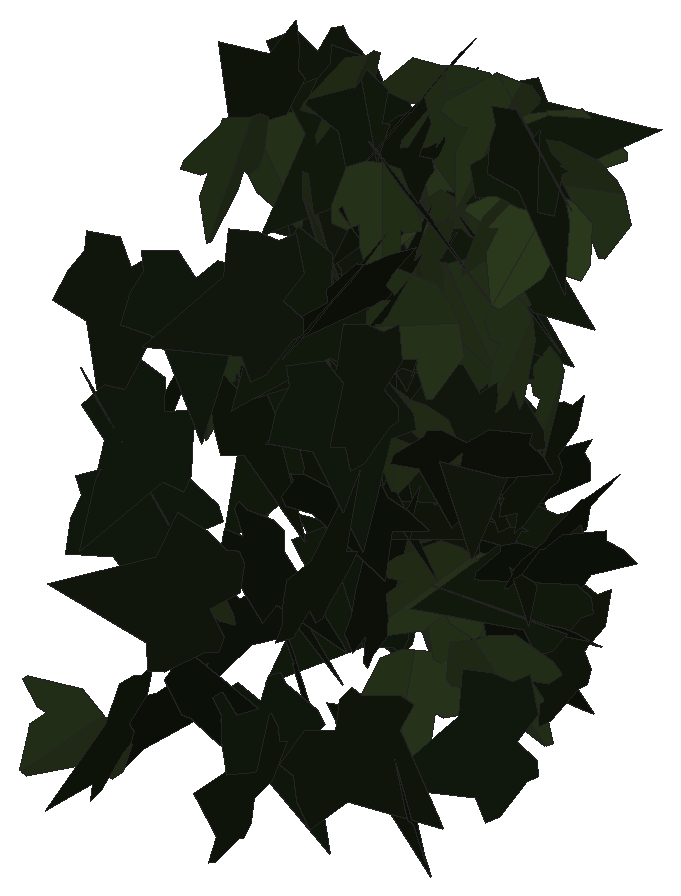
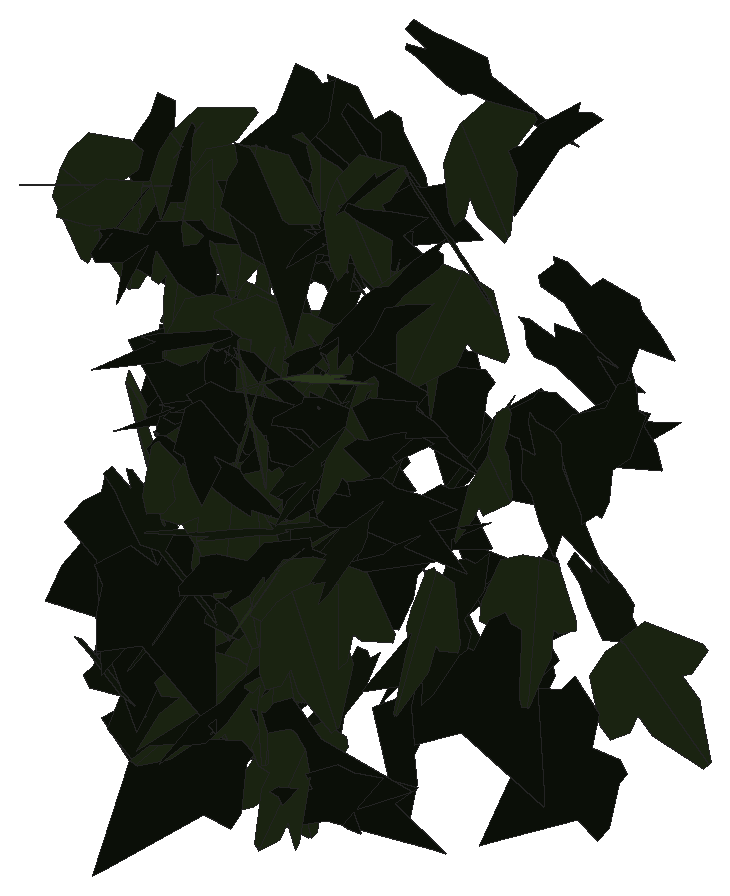
# SketchUp Ruby script. Lengths in inches.
U = 1.inch
M = Sketchup.active_model
def pt(a) = Geom::Point3d.new(a.map { |v| v * U })
def face(e, loops, mat)
  f = e.add_face(loops[0].map { |a| pt(a) })
  loops[1..].each { |l| e.add_face(l.map { |a| pt(a) }).erase! }
  f.material = f.back_material = mat if mat
  f
end
# faces: each face lists its corners as indices into pts; further lists are holes
def faces(e, pts, list, mat = nil) = list.each { |f| face(e, (f[0].is_a?(Array) ? f : [f]).map { |l| l.map { |i| pts[i] } }, mat) }
# xy, xz, yz: faces in a plane at the given z, y or x. An outline is a flat list of corners, or four numbers for a rectangle; further outlines are holes
def ring(l) = l.size == 4 ? [[l[0], l[1]], [l[2], l[1]], [l[2], l[3]], [l[0], l[3]]] : l.each_slice(2).to_a
def flat(e, list, mat, &to3) = list.each { |f| face(e, (f[0].is_a?(Array) ? f : [f]).map { |l| ring(l).map { |u, v| to3.(u, v) } }, mat) }
def xy(e, z, list, mat = nil) = flat(e, list, mat) { |x, y| [x, y, z] }
def xz(e, y, list, mat = nil) = flat(e, list, mat) { |x, z| [x, y, z] }
def yz(e, x, list, mat = nil) = flat(e, list, mat) { |y, z| [x, y, z] }
def lines(e, pts, list) = list.each { |a, b| e.add_line(pt(pts[a]), pt(pts[b])) }
# prism: a flat outline (further loops are holes) pulled along v
def prism(e, loops, v, mat = nil)
  f = face(e, loops, mat); d = Geom::Vector3d.new(v.map { |x| x * U })
  f.pushpull(f.normal.samedirection?(d) ? d.length : -d.length)
end
def box(e, o, s, mat = nil) = prism(e, [[o, [o[0] + s[0], o[1], o[2]], [o[0] + s[0], o[1] + s[1], o[2]], [o[0], o[1] + s[1], o[2]]]], [0, 0, s[2]], mat)
def at(x, y, z, deg = 0) = Geom::Transformation.translation(pt([x, y, z])) * Geom::Transformation.rotation(ORIGIN, Z_AXIS, deg.degrees)
def axes(o, x, y, z) = Geom::Transformation.new([*x, 0, *y, 0, *z, 0, *pt(o).to_a, 1])
def part(name) = M.definitions.add(name)
# library, detail: a bought-in or finely detailed component or shape, given as its bounding box
def library(name, o, s) = part(name).tap { |d| box(d.entities, o, s) }
def detail(e, o, s) = box(e.add_group.entities, o, s)
def put(e, d, t, mat = nil) = e.add_instance(d, t).tap { |i| i.material = mat if mat }
def group(e, t, mat = nil) = e.add_group.tap { |g| g.transformation = t; g.material = mat if mat }.entities
root = M.entities
M.materials.add("efeu1").color = [18, 25, 13]
M.materials.add("efeu2").color = [43, 57, 29]
c1 = part("ivyleaf_9")
p = [[1.54,2.16,1.25],[1.36,2.04,1.19],[-0.21,0.99,0.68],[-0.71,1.11,0.82],[-0.85,0.86,0.67],[-0.8,0.17,0.21],
  [-0.9,-0.01,0.1],[-0.67,-0.16,-0.02],[-0.08,-0.08,-0.05],[-0.03,-0.6,-0.4],[0.65,-0.88,-0.66],[0.83,-0.6,-0.49],
  [1.29,-0.42,-0.43],[1.8125,-0.07,-0.26],[1.21,0.44,0.15]]
faces(c1.entities,p,[[0,1,2,3,4,5,6,7,8,9,10,11,12,13,14]],"efeu1")
c2 = part("ivyleaf_10")
p = [[0,0.5,-0.03],[-0.0625,2.02,-0.43],[-0.19,2.01,-0.46],[-0.54,1.05,-0.29],[-0.52,0.625,-0.18],[-0.83,0.76,-0.28],
  [-1.16,0.64,-0.33],[-1.15,0.33,-0.24],[-0.77,-0.39,0.02],[-0.3,-0.51,0.16],[0.04,-0.48,0.23],[-0.02,2.01,-0.4375],
  [-0.06,2.01,-0.43],[0.04,-0.49,0.23],[0.67,-0.49,0.14],[1.38,0.36,-0.2],[1.375,0.51,-0.24],[0.81,0.65,-0.19],
  [0.62,0.59,-0.15],[0.6,1.09,-0.28],[0.5,1.23,-0.31]]
faces(c2.entities,p,[[0,1,2,3,4,5,6,7,8,9,10],[11,12,0,13,14,15,16,17,18,19,20]],"efeu2")
put(root,c1,axes([49.49,217.875,243.04],[-0.38064,0.31894,-0.05827],[0.04758,-0.03394,-0.49657],[-0.32071,-0.38357,-0.00451]))
put(root,c1,axes([49.97,218.41,244.23],[-0.16811,-0.06264,0.46671],[-0.44313,-0.1466,-0.17929],[0.1593,-0.47391,-0.00622]))
put(root,c1,axes([50.95,218.27,247.84],[-0.4584,0.08446,0.18094],[-0.18201,0.00961,-0.4656],[-0.08212,-0.49272,0.02194]))
put(root,c1,axes([51.67,217.88,245.09],[-0.34679,0.34259,-0.11124],[-0.09527,0.06168,0.48695],[0.34737,0.35893,0.02249]))
put(root,c2,axes([48.75,218.27,242.62],[-0.31441,-0.14442,0.36096],[-0.33345,-0.13853,-0.34587],[0.1999,-0.45821,-0.0092]))
put(root,c1,axes([49.76,218.56,247.46],[-0.01596,-0.49657,-0.05627],[0.00076,0.05628,-0.49682],[0.49974,-0.01594,-0.00105]))
put(root,c1,axes([49.14,218.57,245.05],[-0.20467,-0.31371,-0.33121],[0.17127,0.28362,-0.37447],[0.42282,-0.26674,-0.00864]))
put(root,c1,axes([49.21,218.72,245.82],[-0.47911,-0.08012,-0.11846],[0.11606,0.02412,-0.48574],[0.08355,-0.49295,-0.00452]))
put(root,c1,axes([50.59,218.35,242.47],[-0.26016,0.3656,0.22058],[-0.11707,0.18732,-0.44856],[-0.41062,-0.28504,-0.01187]))
put(root,c1,axes([50.27,218.69,244.89],[0.06676,0.02978,-0.49463],[0.46761,0.16136,0.07283],[0.16396,-0.47231,-0.0063]))
put(root,c1,axes([49.21,218.95,243.04],[0.35299,-0.02966,-0.35287],[0.35202,0.0835,0.34512],[0.03846,-0.49209,0.07983]))
put(root,c1,axes([51.09,219.1,246.5625],[-0.04408,-0.47783,-0.14049],[0.02079,0.13916,-0.4798],[0.49762,-0.04814,0.0076]))
put(root,c1,axes([48.26,219.24,245.17],[0.21386,-0.29811,0.33969],[0.17895,-0.28924,-0.3665],[0.41502,0.27833,-0.01702]))
put(root,c1,axes([51.53,219.03,246.77],[-0.45165,0.18131,0.11463],[-0.10631,0.04287,-0.48668],[-0.18631,-0.46399,-0.00017]))
put(root,c1,axes([50.15,219.07,242.94],[0.20256,-0.43284,-0.14704],[-0.01712,0.15354,-0.47553],[0.45681,0.19768,0.04738]))
put(root,c1,axes([48.44,219.24,246.82],[-0.38996,-0.14618,-0.27671],[0.25876,0.09804,-0.41645],[0.17601,-0.468,-0.00082]))
put(root,c1,axes([51.16,218.92,243.07],[0.06138,-0.20048,-0.45392],[-0.0477,0.45288,-0.20647],[0.49392,0.06865,0.03647]))
put(root,c1,axes([50.95,219.09,247.49],[-0.10512,0.46486,0.15117],[-0.04604,0.14453,-0.47644],[-0.48665,-0.11408,0.01242]))
put(root,c1,axes([50.34,219.75,247.08],[-0.27845,-0.37932,0.16907],[-0.07951,-0.15109,-0.46995],[0.40761,-0.2886,0.02383]))
put(root,c1,axes([48.65,219.06,242.19],[0.17891,0.33436,0.32588],[0.14063,0.29418,-0.37905],[-0.44521,0.22729,0.01122]))
put(root,c1,axes([50.83,219.29,245.33],[0.39725,0.25536,-0.16428],[-0.14598,-0.07658,-0.47204],[-0.26624,0.423,0.01371]))
put(root,c2,axes([48.96,219.43,243.83],[-0.47335,0.0924,0.13192],[-0.12712,0.03716,-0.48214],[-0.0989,-0.48998,-0.01169]))
put(root,c2,axes([49.22,219.88,248.22],[-0.00123,-0.46843,0.17485],[0.05538,-0.1739,-0.4655],[0.49692,0.01823,0.05231]))
put(root,c1,axes([51.01,220.01,242.21],[0.26078,-0.21426,-0.3689],[0.37292,-0.0955,0.31908],[-0.20719,-0.44156,0.10999]))
put(root,c1,axes([48.52,219.88,245.42],[-0.34161,0.21112,-0.29788],[0.25052,-0.16121,-0.40156],[-0.26559,-0.42361,0.00436]))
put(root,c1,axes([50.6875,219.4,247.25],[0.19241,0.40338,0.2242],[0.09865,0.20134,-0.44691],[-0.45083,0.21621,-0.00211]))
put(root,c1,axes([49.16,219.93,243.3],[-0.00601,0.36791,-0.33854],[0.02015,-0.33811,-0.3678],[-0.49956,-0.01806,-0.01076]))
put(root,c1,axes([50.51,220.09,242.32],[0.30092,-0.3908,0.082],[0.05106,-0.06417,-0.49323],[0.39603,0.30521,0.00129]))
put(root,c1,axes([49.05,220.1,245.38],[0.28756,-0.40004,-0.08531],[-0.04857,0.07016,-0.49267],[0.40614,0.29162,0.00149]))
put(root,c2,axes([51.37,220.04,246.97],[0.19411,-0.04289,-0.45878],[-0.44515,0.11112,-0.19873],[0.119,0.48561,0.00495]))
put(root,c1,axes([49.16,220.16,243.75],[0.39867,-0.30079,0.02432],[0.02276,-0.01022,-0.49938],[0.30091,0.39928,0.00554]))
put(root,c2,axes([50.98,220.15,245.84],[-0.46995,-0.07452,0.15359],[-0.15029,-0.03278,-0.47575],[0.08097,-0.49333,0.00841]))
put(root,c1,axes([49.46,220.42,242.47],[0.16434,-0.05251,-0.46929],[0.46214,-0.08423,0.17126],[-0.09705,-0.49005,0.02085]))
put(root,c1,axes([50.8,219.93,246.87],[-0.29195,0.29429,-0.27958],[-0.19467,0.20069,0.41452],[0.35619,0.35088,-0.0026]))
put(root,c2,axes([48.55,220.54,245.69],[-0.06022,0.37894,-0.32059],[0.0226,-0.32051,-0.38309],[-0.49585,-0.06063,0.02148]))
put(root,c1,axes([50.61,220.49,248.02],[0.36771,-0.29598,0.16489],[0.12537,-0.10719,-0.47201],[0.31475,0.38847,-0.00462]))
put(root,c2,axes([50.36,220.47,247.82],[0.47201,-0.0892,0.13875],[0.14156,0.00313,-0.47953],[0.08468,0.49197,0.02821]))
put(root,c2,axes([49.35,220.5,246.63],[-0.35765,0.17722,-0.30112],[0.22877,-0.20694,-0.3935],[-0.2641,-0.41925,0.06694]))
put(root,c1,axes([49.27,220.76,244.96],[-0.25162,-0.41096,0.13339],[-0.0556,-0.12228,-0.48162],[0.42848,-0.25721,0.01584]))
put(root,c1,axes([51.53,220.33,245.62],[0.19496,0.39186,-0.24173],[-0.1457,-0.19652,-0.43607],[-0.43677,0.24047,0.03756]))
put(root,c1,axes([50.51,220.14,243.42],[-0.00156,-0.06042,0.49633],[0.15032,0.47332,0.05809],[-0.47687,0.1494,0.01669]))
put(root,c1,axes([49.51,220.91,246.07],[-0.14521,-0.3463,0.33014],[-0.14085,-0.29878,-0.37536],[0.45725,-0.20201,-0.01078]))
put(root,c2,axes([49.66,220.43,247.34],[-0.3516,0.32795,0.13721],[-0.10113,0.09273,-0.4808],[-0.3408,-0.36586,0.00112]))
put(root,c1,axes([50.1,220.4375,244.86],[-0.1733,-0.22329,0.41244],[0.28804,0.29634,0.28146],[-0.37014,0.33515,0.02592]))
put(root,c1,axes([49.96,220.73,244.89],[0.34291,-0.3518,0.09299],[0.06251,-0.06892,-0.49127],[0.35847,0.34855,-0.00329]))
put(root,c1,axes([51.26,220.84,245.78],[-0.10754,-0.47973,-0.09109],[0.00759,0.09162,-0.49148],[0.48824,-0.10709,-0.01242]))
put(root,c1,axes([51.68,220.79,242.36],[-0.45602,0.08374,0.18718],[-0.18637,0.02114,-0.46349],[-0.08554,-0.49248,0.01193]))
put(root,c2,axes([50.88,220.54,247.15],[-0.17327,0.40518,0.23623],[-0.18998,0.16962,-0.43027],[-0.42882,-0.23886,0.09517]))
put(root,c1,axes([49.07,220.48,246.38],[0.42024,0.25684,0.08623],[0.06004,0.06691,-0.49185],[-0.26419,0.42374,0.02539]))
put(root,c2,axes([50.79,221,243.71],[0.18348,0.26789,-0.38022],[-0.35978,-0.1773,-0.29853],[-0.29477,0.38315,0.1277]))
put(root,c1,axes([50.42,220.95,247.97],[-0.45146,0.18374,-0.11144],[0.10413,-0.03979,-0.48742],[-0.18798,-0.46331,-0.00234]))
put(root,c1,axes([49.56,221.26,245.78],[-0.11597,-0.41918,0.24665],[0.27254,-0.26602,-0.32396],[0.40283,0.05931,0.29019]))
put(root,c1,axes([49.03,221.29,244.96],[-0.23633,-0.4291,0.1001],[0.06334,-0.14549,-0.47415],[0.43605,-0.21143,0.12312]))
put(root,c2,axes([51.58,221.01,246.49],[0.38026,-0.30291,-0.11683],[-0.09341,0.07024,-0.48615],[0.31093,0.39155,-0.00318]))
put(root,c2,axes([50.28,221.07,242.41],[0.19305,0.43669,-0.14843],[-0.05435,-0.13825,-0.47742],[-0.45802,0.20047,-0.00591]))
put(root,c1,axes([49.75,221.28,245.63],[0.06648,-0.46985,0.15754],[0.04372,-0.15277,-0.47408],[0.49363,0.0768,0.02077]))
put(root,c1,axes([49.68,221.3125,247.89],[-0.40798,-0.26287,0.12023],[-0.08611,-0.088,-0.4846],[0.27594,-0.41612,0.02653]))
put(root,c1,axes([49.74,221.37,246.68],[-0.19463,-0.02071,0.4601],[0.02256,-0.49932,-0.01293],[0.46001,0.01573,0.1953]))
put(root,c1,axes([48.8125,220.78,247.94],[-0.12675,0.28627,0.38985],[-0.22222,0.32349,-0.3098],[-0.4296,-0.2518,0.04523]))
put(root,c2,axes([48.89,220.86,244.35],[0.07554,-0.37189,-0.32557],[0.04043,0.33289,-0.37088],[0.4926,0.0297,0.08036]))
put(root,c2,axes([48.58,221.05,247.51],[-0.45157,-0.13962,-0.16308],[0.17517,-0.02007,-0.46788],[0.1241,-0.47969,0.06704]))
put(root,c1,axes([50.76,221.49,244.05],[-0.45065,-0.20047,0.08201],[0.16879,-0.44367,-0.15705],[0.13574,-0.11387,0.46756]))
put(root,c1,axes([49.45,221.27,246.53],[-0.49222,-0.02983,0.08266],[-0.08323,0.00729,-0.49297],[0.02821,-0.49906,-0.01214]))
put(root,c2,axes([49.38,221.36,248.28],[0.04995,-0.47015,0.16267],[0.03972,-0.1592,-0.47231],[0.49591,0.06011,0.02144]))
put(root,c2,axes([51.1875,221.11,242.93],[-0.45416,-0.03977,-0.20531],[0.20281,0.03602,-0.4556],[0.05103,-0.49711,-0.01659]))
put(root,c2,axes([51.45,221.57,247.4375],[-0.46436,-0.11683,0.14396],[0.07859,-0.47567,-0.13253],[0.16792,-0.10045,0.46012]))
put(root,c1,axes([49.49,221.51,248.09],[0.01985,-0.48833,0.10553],[-0.01193,-0.10605,-0.48848],[0.49946,0.01688,-0.01587]))
put(root,c2,axes([50.74,221.2,246.68],[-0.46669,-0.12285,-0.13078],[0.13154,0.01363,-0.4822],[0.12204,-0.48448,0.0196]))
put(root,c1,axes([49.63,221.58,246.08],[-0.1408,-0.46699,-0.10998],[0.02314,0.10788,-0.48768],[0.47921,-0.14242,-0.00877]))
put(root,c2,axes([50.9,221.6875,248.37],[-0.08829,-0.39512,0.2934],[0.0463,-0.30343,-0.3947],[0.48996,-0.04253,0.09017]))
put(root,c2,axes([50.16,221.33,243.69],[-0.0118,-0.46172,-0.19151],[0.02658,0.19071,-0.46144],[0.49915,-0.02107,0.02004]))
put(root,c1,axes([51.46,221.78,243.59],[-0.31079,-0.135,0.36767],[-0.27697,-0.25613,-0.32816],[0.27694,-0.40765,0.08443]))
put(root,c1,axes([51.47,221.79,242.97],[-0.49903,-0.02112,0.02298],[0.02311,-0.49747,0.0446],[0.02098,0.04557,0.49748]))
put(root,c1,axes([49.2,221.82,247.19],[-0.2375,-0.42068,0.12894],[-0.05123,-0.1191,-0.4829],[0.437,-0.24259,0.01347]))
put(root,c1,axes([49.55,221.68,244.29],[0.2779,-0.41154,0.05836],[0.02654,-0.05249,-0.49653],[0.41481,0.27906,-0.00733]))
put(root,c1,axes([51.19,221.75,248.05],[0.15779,-0.47121,0.05533],[0.01218,-0.05427,-0.4969],[0.47429,0.15816,-0.00565]))
put(root,c1,axes([51.59,221.4,244.05],[0.20555,0.42822,-0.15612],[-0.09228,-0.12862,-0.47428],[-0.44636,0.22379,0.02616]))
put(root,c1,axes([48.94,221.84,245.76],[-0.44525,-0.22624,0.02377],[-0.00901,-0.03468,-0.49871],[0.22731,-0.44454,0.0268]))
put(root,c2,axes([51.49,221.61,245.63],[0.32703,-0.36827,-0.08621],[-0.04838,0.07231,-0.49237],[0.37512,0.33038,0.01166]))
put(root,c2,axes([51.05,221.5,247.44],[0.00713,-0.45882,-0.19858],[0.04021,0.19848,-0.45715],[0.49833,-0.00945,0.03973]))
put(root,c1,axes([49.31,221.88,242.8],[-0.43627,-0.2233,0.099],[-0.07593,-0.06864,-0.48941],[0.23216,-0.44207,0.02598]))
put(root,c2,axes([50.46,221.68,248.23],[-0.12544,-0.48398,0.00548],[0.0382,-0.01555,-0.4983],[0.4825,-0.1246,0.04087]))
put(root,c1,axes([51.82,221.61,243],[-0.39449,0.28356,0.1182],[-0.11495,0.04215,-0.48478],[-0.28489,-0.40966,0.03193]))
put(root,c1,axes([49.13,222.02,246],[-0.23154,-0.40705,0.17523],[-0.06952,-0.16189,-0.46793],[0.43767,-0.24105,0.01837]))
put(root,c1,axes([50.26,221.57,247.97],[-0.31823,0.38201,0.05291],[-0.02837,0.04522,-0.49714],[-0.38461,-0.31942,-0.0071]))
put(root,c2,axes([50.59,221.53,243.1875],[-0.20971,-0.26377,-0.36939],[0.32933,0.19159,-0.32378],[0.31235,-0.3791,0.09338]))
put(root,c2,axes([49.71,221.91,244.78],[-0.09663,-0.43411,0.22849],[0.38919,-0.20961,-0.23365],[0.29865,0.1327,0.37841]))
put(root,c1,axes([49.74,221.61,242.78],[-0.1412,0.1148,0.46571],[-0.38619,0.2607,-0.18136],[-0.28446,-0.41092,0.01505]))
put(root,c1,axes([51.65,221.35,244.22],[0.05219,0.44631,0.21928],[0.00515,0.21999,-0.44898],[-0.49724,0.04912,0.01836]))
put(root,c2,axes([50.24,221.68,248.38],[-0.47526,-0.15531,-0.00178],[0.00301,-0.00346,-0.49998],[0.15529,-0.47525,0.00422]))
put(root,c1,axes([50.75,222.01,244.15],[0.1224,-0.44655,0.1887],[0.04484,-0.18336,-0.463],[0.48271,0.13027,-0.00484]))
put(root,c1,axes([51.44,221.71,244.86],[-0.38065,0.32417,0.00399],[-0.013,-0.00912,-0.49975],[-0.32394,-0.38056,0.01537]))
put(root,c1,axes([50.04,221.48,248.21],[-0.0922,0.47515,0.12544],[-0.03134,0.12168,-0.48395],[-0.49043,-0.0971,0.00735]))
put(root,c2,axes([48.91,221.98,246.47],[-0.02428,0.36028,-0.34584],[-0.01135,-0.34656,-0.36023],[-0.49928,-0.00964,0.02501]))
put(root,c1,axes([51.15,221.6,248.38],[0.38411,-0.03997,-0.31759],[-0.31072,0.07263,-0.38494],[0.0769,0.49308,0.03095]))
put(root,c1,axes([48.82,221.87,245.57],[0.32348,-0.38096,0.01528],[0.00405,-0.01661,-0.49971],[0.38124,0.32341,-0.00767]))
put(root,c1,axes([48.56,221.88,247.97],[0.12995,-0.46544,-0.12837],[-0.01673,0.12851,-0.48291],[0.48253,0.12981,0.01782]))
put(root,c1,axes([48.89,221.98,246.7],[-0.22486,-0.39947,-0.19966],[0.17571,0.12637,-0.45073],[0.41057,-0.27286,0.08355]))
put(root,c2,axes([49.43,222.18,246.88],[-0.4647,-0.14435,0.11495],[0.13018,-0.4772,-0.07301],[0.13078,-0.03793,0.4811]))
put(root,c2,axes([50.38,221.73,244.92],[-0.40518,0.06165,0.28641],[-0.28381,0.03862,-0.40983],[-0.07265,-0.49468,0.0037]))
put(root,c1,axes([50.42,222.01,246.57],[0.24829,-0.3241,0.28864],[0.20303,-0.20717,-0.40726],[0.38358,0.31944,0.02873]))
put(root,c2,axes([50.64,221.9,245.65],[-0.2162,-0.44718,0.05732],[-0.03269,-0.04785,-0.49663],[0.44965,-0.21849,-0.00854]))
put(root,c1,axes([49.97,221.98,246.72],[-0.49881,0.03396,-0.00564],[0.00561,-0.00052,-0.49997],[-0.03396,-0.49885,0.00013]))
put(root,c2,axes([51.92,221.78,247.78],[0.14897,0.07031,-0.47209],[-0.45647,0.16547,-0.1194],[0.13944,0.46656,0.11348]))
put(root,c2,axes([50.4,221.81,246.91],[-0.4949,-0.02355,0.06726],[-0.06664,-0.01442,-0.49533],[0.02527,-0.49924,0.01113]))
put(root,c1,axes([50.375,221.8,246.8],[0.20957,-0.34828,-0.29117],[0.2199,0.35845,-0.27047],[0.39714,-0.01469,0.30342]))
put(root,c2,axes([50.29,221.85,245.46],[-0.43757,-0.24193,-0.00195],[0.0008,0.00259,-0.49999],[0.24194,-0.43756,-0.00188]))
put(root,c2,axes([49.63,221.88,242.91],[-0.38622,0.27409,-0.16034],[0.1183,-0.1101,-0.47316],[-0.29469,-0.40342,0.0202]))
put(root,c2,axes([49.28,221.85,244.75],[-0.46957,-0.16462,-0.04907],[0.04983,0.00613,-0.49747],[0.16439,-0.47208,0.01065]))
put(root,c1,axes([50.92,221.6,248.03],[0.46706,-0.10141,-0.14687],[0.06289,0.47857,-0.13046],[0.16703,0.10339,0.45979]))
put(root,c1,axes([49.9,222.09,244.91],[-0.24982,-0.41476,-0.12474],[0.06861,0.10429,-0.48417],[0.42765,-0.25903,0.00481]))
put(root,c1,axes([49.07,222.06,246.27],[0.26272,-0.41828,0.07759],[0.04754,-0.06175,-0.49389],[0.42275,0.26688,0.00732]))
put(root,c1,axes([50.11,221.88,246.32],[0.21013,-0.36937,-0.26346],[0.22047,0.33688,-0.29649],[0.39654,0.00843,0.30445]))
put(root,c2,axes([49.58,221.94,247.25],[0.46055,0.16083,0.10968],[0.10165,0.04159,-0.48779],[-0.16602,0.4716,0.00561]))
put(root,c1,axes([50.72,221.7,242.69],[0.44536,0.22603,0.02376],[0.017,0.019,-0.49935],[-0.22664,0.44559,0.00924]))
put(root,c1,axes([50.89,222.19,247.78],[-0.35276,-0.34599,-0.07648],[0.08009,0.02727,-0.49279],[0.34517,-0.35993,0.03618]))
put(root,c1,axes([49.73,221.9,245.22],[0.29918,-0.37008,-0.1534],[0.24403,0.32018,-0.29653],[0.31771,0.10257,0.37221]))
put(root,c1,axes([50.41,222.16,245.75],[-0.40955,-0.17806,-0.22486],[0.22776,0.03638,-0.44363],[0.17434,-0.4658,0.05131]))
put(root,c1,axes([50.09,222.24,243.54],[0.05021,-0.49503,0.04924],[0.01587,-0.04787,-0.49745],[0.49722,0.05152,0.0109]))
put(root,c2,axes([49.92,221.88,246.73],[-0.29474,0.40009,0.05528],[-0.02075,0.05334,-0.49671],[-0.40336,-0.29509,-0.01484]))
put(root,c1,axes([50.18,222.29,246.49],[-0.12257,0.0938,-0.47558],[0.29903,-0.37146,-0.15033],[-0.38152,-0.32128,0.03497]))
put(root,c2,axes([51.16,221.99,247.97],[0.34838,0.35598,0.04369],[0.0393,0.02266,-0.49794],[-0.35649,0.35038,-0.01219]))
put(root,c1,axes([50.96,221.99,244.4],[-0.05555,0.43103,-0.24724],[0.01995,-0.24664,-0.43448],[-0.4965,-0.05814,0.0102]))
put(root,c1,axes([50.21,222.27,246.33],[-0.45126,-0.13354,0.16892],[-0.16219,-0.04721,-0.4706],[0.14163,-0.47952,-0.00071]))
put(root,c2,axes([49.95,222.04,246.75],[0.22039,-0.43922,-0.09226],[-0.03061,0.08783,-0.49127],[0.44776,0.22219,0.01183]))
put(root,c2,axes([49.28,222.14,244.58],[-0.14518,-0.46689,0.10459],[-0.04815,-0.09449,-0.48862],[0.47603,-0.15194,-0.01752]))
